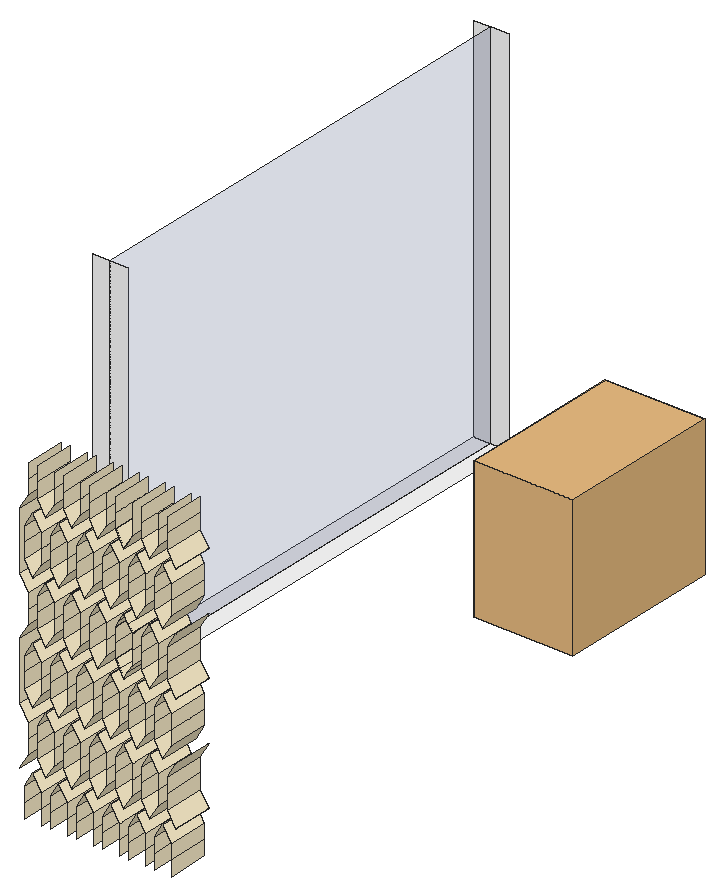
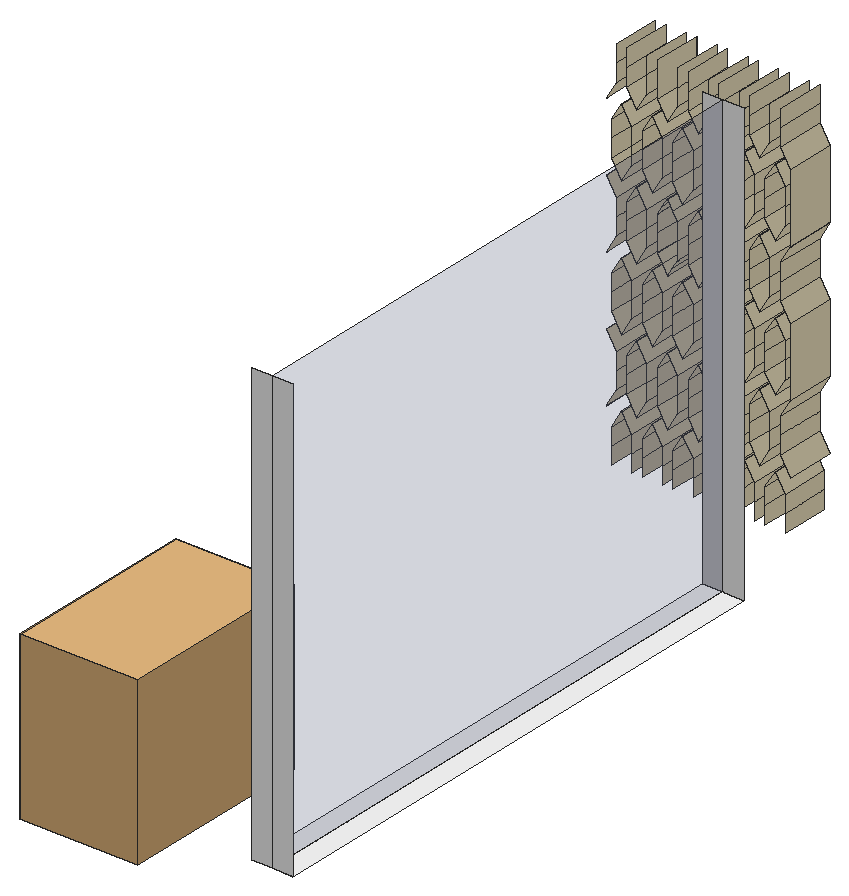
# SketchUp Ruby script. Lengths in inches.
U = 1.inch
M = Sketchup.active_model
def pt(a) = Geom::Point3d.new(a.map { |v| v * U })
def face(e, loops, mat)
  f = e.add_face(loops[0].map { |a| pt(a) })
  loops[1..].each { |l| e.add_face(l.map { |a| pt(a) }).erase! }
  f.material = f.back_material = mat if mat
  f
end
# faces: each face lists its corners as indices into pts; further lists are holes
def faces(e, pts, list, mat = nil) = list.each { |f| face(e, (f[0].is_a?(Array) ? f : [f]).map { |l| l.map { |i| pts[i] } }, mat) }
# xy, xz, yz: faces in a plane at the given z, y or x. An outline is a flat list of corners, or four numbers for a rectangle; further outlines are holes
def ring(l) = l.size == 4 ? [[l[0], l[1]], [l[2], l[1]], [l[2], l[3]], [l[0], l[3]]] : l.each_slice(2).to_a
def flat(e, list, mat, &to3) = list.each { |f| face(e, (f[0].is_a?(Array) ? f : [f]).map { |l| ring(l).map { |u, v| to3.(u, v) } }, mat) }
def xy(e, z, list, mat = nil) = flat(e, list, mat) { |x, y| [x, y, z] }
def xz(e, y, list, mat = nil) = flat(e, list, mat) { |x, z| [x, y, z] }
def yz(e, x, list, mat = nil) = flat(e, list, mat) { |y, z| [x, y, z] }
def lines(e, pts, list) = list.each { |a, b| e.add_line(pt(pts[a]), pt(pts[b])) }
# prism: a flat outline (further loops are holes) pulled along v
def prism(e, loops, v, mat = nil)
  f = face(e, loops, mat); d = Geom::Vector3d.new(v.map { |x| x * U })
  f.pushpull(f.normal.samedirection?(d) ? d.length : -d.length)
end
def box(e, o, s, mat = nil) = prism(e, [[o, [o[0] + s[0], o[1], o[2]], [o[0] + s[0], o[1] + s[1], o[2]], [o[0], o[1] + s[1], o[2]]]], [0, 0, s[2]], mat)
def at(x, y, z, deg = 0) = Geom::Transformation.translation(pt([x, y, z])) * Geom::Transformation.rotation(ORIGIN, Z_AXIS, deg.degrees)
def axes(o, x, y, z) = Geom::Transformation.new([*x, 0, *y, 0, *z, 0, *pt(o).to_a, 1])
def part(name) = M.definitions.add(name)
# library, detail: a bought-in or finely detailed component or shape, given as its bounding box
def library(name, o, s) = part(name).tap { |d| box(d.entities, o, s) }
def detail(e, o, s) = box(e.add_group.entities, o, s)
def put(e, d, t, mat = nil) = e.add_instance(d, t).tap { |i| i.material = mat if mat }
def group(e, t, mat = nil) = e.add_group.tap { |g| g.transformation = t; g.material = mat if mat }.entities
root = M.entities
M.materials.add("D01_Frost_White").color = [255, 242, 206]
M.materials.add("Glass_Sky Reflection_01").color = [126, 138, 183]
M.materials["Glass_Sky Reflection_01"].alpha = 0.25
M.materials.add("M00_Soft_Cloud").color = [255, 255, 255]
c1 = library("FF_Model_ID8636_1_ruthrocker1",[-22.29,-12.06,-2.32],[42.44,25.59,36.01])
xy(root,149.0192,[[126,153.6841,130.5,276.2837],[130.5,153.6841,135,276.2837]],"M00_Soft_Cloud")
xy(root,197.0101,[[183.1657,109.0676,183.1728,119.6039]],"D01_Frost_White")
xy(root,197.0223,[[163.0893,109.0676,163.0964,119.6039],[169.7802,109.0676,169.7874,119.6039]],"D01_Frost_White")
xz(root,109.0676,[[169.7874,182.0245,169.7909,182.0306,168.6907,183.8901],[169.7945,182.0245,170.8947,183.9084,169.7909,182.0306],[168.6907,183.8901,167.5869,185.7679,167.5869,185.7557],[170.8947,183.9084,171.9914,185.774,171.9914,185.7861],[167.5869,185.7679,167.5833,189.5052,167.5833,185.774],
  [171.9914,185.7861,171.995,185.7922,171.9914,189.5416],[167.5833,189.5052,167.5833,193.2607,167.5797,193.2546],[171.9914,189.5416,171.9914,193.2728,171.9879,193.2789],[167.5833,193.2607,168.68,195.1384,167.5833,193.2728],[171.9879,193.2789,171.9878,193.2911,170.884,195.1567],
  [168.68,195.1384,169.7838,197.0162,169.7802,197.0223],[170.884,195.1567,169.7909,197.0162,169.7909,197.0163,169.7874,197.0223,169.7838,197.0162],[183.1639,197.0101,183.1657,197.0101,183.1656,197.0102,183.1639,197.0132],[169.7838,197.0162,169.7874,197.0223,169.7802,197.0223],[143.0236,197.0223,143.0271,197.0224,143.0236,197.0283],
  [143.0236,197.0223,143.0272,197.0223,143.0271,197.0224],[149.711,197.0223,149.7181,197.0223,149.7162,197.0256,149.7129,197.0256],[156.4019,197.0223,156.4055,197.0223,156.4054,197.0224,156.4037,197.0253],[156.4055,197.0223,156.4055,197.0283,156.4037,197.0253,156.4054,197.0224],[149.7129,197.0256,149.7162,197.0256,149.7146,197.0283],
  [183.1639,212.0169,183.1675,212.023,183.1639,212.0291],[169.7802,212.0321,167.5797,215.7876,167.5797,215.7755],[167.5797,215.7876,167.5833,223.2804,167.5797,223.2743]],"D01_Frost_White")
xz(root,153.6841,[[126,149.0192,130.5,245.0192],[130.5,149.0192,135,245.0192]],"M00_Soft_Cloud")
xz(root,276.2837,[[126,149.0192,130.5,245.0192],[130.5,149.0192,135,245.0192]],"M00_Soft_Cloud")
yz(root,130.5,[[153.6841,149.0192,276.2837,245.0192]],"Glass_Sky Reflection_01")
yz(root,143.0236,[[109.0676,167.0329,119.6039,182.0306],[109.0676,197.0283,119.6039,212.0261]],"D01_Frost_White")
yz(root,144.165,[[109.0676,140.7869,119.6039,144.5363],[109.0676,144.5363,119.6039,148.2857],[109.0676,170.7823,119.6039,174.5318],[109.0676,174.5318,119.6039,178.2812],[109.0676,200.7778,119.6039,204.5272],
  [109.0676,204.5272,119.6039,208.2766]],"D01_Frost_White")
yz(root,145.2277,[[109.0676,155.7846,119.6039,159.534],[109.0676,159.534,119.6039,163.2835],[109.0676,185.78,119.6039,189.5295],[109.0676,189.5295,119.6039,193.2789],[109.0676,215.7755,119.6039,219.5249],
  [109.0676,219.5249,119.6039,223.2743]],"D01_Frost_White")
yz(root,147.5105,[[109.0676,155.7846,119.6039,159.534],[109.0676,159.534,119.6039,163.2835],[109.0676,185.78,119.6039,189.5295],[109.0676,189.5295,119.6039,193.2789],[109.0676,215.7755,119.6039,219.5249],
  [109.0676,219.5249,119.6039,223.2743]],"D01_Frost_White")
yz(root,148.5731,[[109.0676,140.7869,119.6039,144.5363],[109.0676,144.5363,119.6039,148.2857],[109.0676,170.7823,119.6039,174.5318],[109.0676,174.5318,119.6039,178.2812],[109.0676,200.7778,119.6039,204.5272],
  [109.0676,204.5272,119.6039,208.2766]],"D01_Frost_White")
yz(root,150.856,[[109.0676,140.7869,119.6039,144.5363],[109.0676,144.5363,119.6039,148.2857],[109.0676,170.7823,119.6039,174.5318],[109.0676,174.5318,119.6039,178.2812],[109.0676,200.7778,119.6039,204.5272],
  [109.0676,204.5272,119.6039,208.2766]],"D01_Frost_White")
yz(root,151.9186,[[109.0676,155.7846,119.6039,159.534],[109.0676,159.534,119.6039,163.2835],[109.0676,185.78,119.6039,189.5295],[109.0676,189.5295,119.6039,193.2789],[109.0676,215.7755,119.6039,219.5249],
  [109.0676,219.5249,119.6039,223.2743]],"D01_Frost_White")
yz(root,154.2015,[[109.0676,155.7846,119.6039,159.534],[109.0676,159.534,119.6039,163.2835],[109.0676,185.78,119.6039,189.5295],[109.0676,189.5295,119.6039,193.2789],[109.0676,215.7755,119.6039,219.5249],
  [109.0676,219.5249,119.6039,223.2743]],"D01_Frost_White")
yz(root,155.2641,[[109.0676,140.7869,119.6039,144.5363],[109.0676,144.5363,119.6039,148.2857],[109.0676,170.7823,119.6039,174.5318],[109.0676,174.5318,119.6039,178.2812],[109.0676,200.7778,119.6039,204.5272],
  [109.0676,204.5272,119.6039,208.2766]],"D01_Frost_White")
yz(root,156.4055,[[109.0676,152.0291,119.6039,152.0352],[109.0676,167.0268,119.6039,167.0329],[109.0676,182.0245,119.6039,182.0306],[109.0676,197.0223,119.6039,197.0283]],"D01_Frost_White")
yz(root,157.5433,[[109.0676,200.7778,119.6039,204.5272],[109.0676,204.5272,119.6039,208.2766]],"D01_Frost_White")
yz(root,157.5469,[[109.0676,140.7808,119.6039,144.5302],[109.0676,144.5302,119.6039,148.2797],[109.0676,170.7762,119.6039,174.5257],[109.0676,174.5257,119.6039,178.2751]],"D01_Frost_White")
yz(root,158.606,[[109.0676,215.7755,119.6039,219.5249],[109.0676,219.5249,119.6039,223.2743]],"D01_Frost_White")
yz(root,158.6095,[[109.0676,155.7785,119.6039,159.528],[109.0676,159.528,119.6039,163.2774],[109.0676,185.774,119.6039,189.5234],[109.0676,189.5234,119.6039,193.2728]],"D01_Frost_White")
yz(root,160.8888,[[109.0676,215.7755,119.6039,219.5249],[109.0676,219.5249,119.6039,223.2743]],"D01_Frost_White")
yz(root,160.8924,[[109.0676,155.7785,119.6039,159.528],[109.0676,159.528,119.6039,163.2774],[109.0676,185.774,119.6039,189.5234],[109.0676,189.5234,119.6039,193.2728]],"D01_Frost_White")
yz(root,161.9514,[[109.0676,200.7778,119.6039,204.5272],[109.0676,204.5272,119.6039,208.2766]],"D01_Frost_White")
yz(root,161.955,[[109.0676,140.7808,119.6039,144.5302],[109.0676,144.5302,119.6039,148.2797],[109.0676,170.7762,119.6039,174.5257],[109.0676,174.5257,119.6039,178.2751]],"D01_Frost_White")
yz(root,164.2343,[[109.0676,200.7778,119.6039,204.5272],[109.0676,204.5272,119.6039,208.2766]],"D01_Frost_White")
yz(root,164.2379,[[109.0676,140.7808,119.6039,144.5302],[109.0676,144.5302,119.6039,148.2797],[109.0676,170.7762,119.6039,174.5257],[109.0676,174.5257,119.6039,178.2751]],"D01_Frost_White")
yz(root,165.2969,[[109.0676,215.7755,119.6039,219.5249],[109.0676,219.5249,119.6039,223.2743]],"D01_Frost_White")
yz(root,165.3005,[[109.0676,155.7785,119.6039,159.528],[109.0676,159.528,119.6039,163.2774],[109.0676,185.774,119.6039,189.5234],[109.0676,189.5234,119.6039,193.2728]],"D01_Frost_White")
yz(root,167.5797,[[109.0676,215.7755,119.6039,215.7876],[109.0676,215.7876,119.6039,219.5249],[109.0676,219.5249,119.6039,223.2743]],"D01_Frost_White")
yz(root,167.5833,[[109.0676,155.7785,119.6039,159.528],[109.0676,159.528,119.6039,163.2774],[109.0676,185.774,119.6039,189.5052],[109.0676,193.2607,119.6039,193.2728]],"D01_Frost_White")
yz(root,167.5869,[[109.0676,185.7557,119.6039,185.7679]],"D01_Frost_White")
yz(root,168.6424,[[109.0676,200.7778,119.6039,204.5272],[109.0676,204.5272,119.6039,208.2766]],"D01_Frost_White")
yz(root,168.6459,[[109.0676,140.7808,119.6039,144.5302],[109.0676,144.5302,119.6039,148.2797],[109.0676,170.7762,119.6039,174.5257],[109.0676,174.5257,119.6039,178.2751]],"D01_Frost_White")
yz(root,169.7909,[[109.0676,197.0162,119.6039,197.0163]],"D01_Frost_White")
yz(root,170.9288,[[109.0676,140.7808,119.6039,144.5302],[109.0676,144.5302,119.6039,148.2797],[109.0676,170.7762,119.6039,174.5257],[109.0676,174.5257,119.6039,178.2751],[109.0676,200.7717,119.6039,204.5211],
  [109.0676,204.5211,119.6039,208.2706]],"D01_Frost_White")
yz(root,171.9914,[[109.0676,155.7785,119.6039,159.528],[109.0676,159.528,119.6039,163.2774],[109.0676,185.774,119.6039,185.7861],[109.0676,189.5416,119.6039,193.2728]],"D01_Frost_White")
yz(root,174.2743,[[109.0676,155.7785,119.6039,159.528],[109.0676,159.528,119.6039,163.2774],[109.0676,185.774,119.6039,189.5234],[109.0676,189.5234,119.6039,193.2728],[109.0676,215.7694,119.6039,219.5188],
  [109.0676,219.5188,119.6039,223.2683]],"D01_Frost_White")
yz(root,175.3369,[[109.0676,140.7808,119.6039,144.5302],[109.0676,144.5302,119.6039,148.2797],[109.0676,170.7762,119.6039,174.5257],[109.0676,174.5257,119.6039,178.2751],[109.0676,200.7717,119.6039,204.5211],
  [109.0676,204.5211,119.6039,208.2706]],"D01_Frost_White")
yz(root,177.6197,[[109.0676,140.7808,119.6039,144.5302],[109.0676,144.5302,119.6039,148.2797],[109.0676,170.7762,119.6039,174.5257],[109.0676,174.5257,119.6039,178.2751],[109.0676,200.7717,119.6039,204.5211],
  [109.0676,204.5211,119.6039,208.2706]],"D01_Frost_White")
yz(root,178.6824,[[109.0676,155.7785,119.6039,159.528],[109.0676,159.528,119.6039,163.2774],[109.0676,185.774,119.6039,189.5234],[109.0676,189.5234,119.6039,193.2728],[109.0676,215.7694,119.6039,219.5188],
  [109.0676,219.5188,119.6039,223.2683]],"D01_Frost_White")
yz(root,180.9652,[[109.0676,155.7785,119.6039,159.528],[109.0676,159.528,119.6039,163.2774],[109.0676,185.774,119.6039,189.5234],[109.0676,189.5234,119.6039,193.2728],[109.0676,215.7694,119.6039,219.5188],
  [109.0676,219.5188,119.6039,223.2683]],"D01_Frost_White")
yz(root,182.0278,[[109.0676,140.7808,119.6039,144.5302],[109.0676,144.5302,119.6039,148.2797],[109.0676,170.7762,119.6039,174.5257],[109.0676,174.5257,119.6039,178.2751],[109.0676,200.7717,119.6039,204.5211],
  [109.0676,204.5211,119.6039,208.2706]],"D01_Frost_White")
yz(root,183.1639,[[109.0676,212.0169,119.6039,212.0291]],"D01_Frost_White")
yz(root,183.1692,[[109.0676,152.023,119.6039,152.0291],[109.0676,167.0207,119.6039,167.0268],[109.0676,182.0185,119.6039,182.0245]],"D01_Frost_White")
p = [[144.165,109.0676,148.2857],[146.3691,109.0676,152.0352],[146.3691,119.6039,152.0352],[144.165,119.6039,148.2857],[148.5731,109.0676,148.2857],[148.5731,119.6039,148.2857],
  [150.856,109.0676,148.2857],[153.06,109.0676,152.0352],[153.06,119.6039,152.0352],[150.856,119.6039,148.2857],[155.2641,109.0676,148.2857],[155.2641,119.6039,148.2857],
  [157.5469,109.0676,148.2797],[159.751,109.0676,152.0291],[159.751,119.6039,152.0291],[157.5469,119.6039,148.2797],[161.955,109.0676,148.2797],[161.955,119.6039,148.2797],
  [164.2379,109.0676,148.2797],[166.4419,109.0676,152.0291],[166.4419,119.6039,152.0291],[164.2379,119.6039,148.2797],[168.6459,109.0676,148.2797],[168.6459,119.6039,148.2797],
  [170.9288,109.0676,148.2797],[173.1328,109.0676,152.0291],[173.1328,119.6039,152.0291],[170.9288,119.6039,148.2797],[175.3369,109.0676,148.2797],[175.3369,119.6039,148.2797],
  [177.6197,109.0676,148.2797],[179.8238,109.0676,152.0291],[179.8238,119.6039,152.0291],[177.6197,119.6039,148.2797],[182.0278,109.0676,148.2797],[182.0278,119.6039,148.2797],
  [145.2277,109.0676,155.7846],[143.0236,109.0676,152.0352],[143.0236,119.6039,152.0352],[145.2277,119.6039,155.7846],[149.7146,109.0676,152.0352],[147.5105,109.0676,155.7846],
  [147.5105,119.6039,155.7846],[149.7146,119.6039,152.0352],[151.9186,109.0676,155.7846],[151.9186,119.6039,155.7846],[156.4055,109.0676,152.0352],[154.2015,109.0676,155.7846],
  [154.2015,119.6039,155.7846],[156.4055,119.6039,152.0352],[158.6095,109.0676,155.7785],[156.4055,109.0676,152.0291],[156.4055,119.6039,152.0291],[158.6095,119.6039,155.7785],
  [163.0964,109.0676,152.0291],[160.8924,109.0676,155.7785],[160.8924,119.6039,155.7785],[163.0964,119.6039,152.0291],[165.3005,109.0676,155.7785],[165.3005,119.6039,155.7785],
  [169.7874,109.0676,152.0291],[167.5833,109.0676,155.7785],[167.5833,119.6039,155.7785],[169.7874,119.6039,152.0291],[171.9914,109.0676,155.7785],[171.9914,119.6039,155.7785],
  [176.4783,109.0676,152.0291],[174.2743,109.0676,155.7785],[174.2743,119.6039,155.7785],[176.4783,119.6039,152.0291],[178.6824,109.0676,155.7785],[178.6824,119.6039,155.7785],
  [183.1692,109.0676,152.0291],[180.9652,109.0676,155.7785],[180.9652,119.6039,155.7785],[183.1692,119.6039,152.0291],[143.0236,109.0676,167.0329],[145.2277,109.0676,163.2835],
  [145.2277,119.6039,163.2835],[143.0236,119.6039,167.0329],[147.5105,109.0676,163.2835],[149.7146,109.0676,167.0329],[149.7146,119.6039,167.0329],[147.5105,119.6039,163.2835],
  [151.9186,109.0676,163.2835],[151.9186,119.6039,163.2835],[154.2015,109.0676,163.2835],[156.4055,109.0676,167.0329],[156.4055,119.6039,167.0329],[154.2015,119.6039,163.2835],
  [156.4055,109.0676,167.0268],[158.6095,109.0676,163.2774],[158.6095,119.6039,163.2774],[156.4055,119.6039,167.0268],[160.8924,109.0676,163.2774],[163.0964,109.0676,167.0268],
  [163.0964,119.6039,167.0268],[160.8924,119.6039,163.2774],[165.3005,109.0676,163.2774],[165.3005,119.6039,163.2774],[167.5833,109.0676,163.2774],[169.7874,109.0676,167.0268],
  [169.7874,119.6039,167.0268],[167.5833,119.6039,163.2774],[171.9914,109.0676,163.2774],[171.9914,119.6039,163.2774],[174.2743,109.0676,163.2774],[176.4783,109.0676,167.0268],
  [176.4783,119.6039,167.0268],[174.2743,119.6039,163.2774],[178.6824,109.0676,163.2774],[178.6824,119.6039,163.2774],[180.9652,109.0676,163.2774],[183.1692,109.0676,167.0268],
  [183.1692,119.6039,167.0268],[180.9652,119.6039,163.2774],[146.3691,109.0676,167.0329],[144.165,109.0676,170.7823],[144.165,119.6039,170.7823],[146.3691,119.6039,167.0329],
  [148.5731,109.0676,170.7823],[148.5731,119.6039,170.7823],[153.06,109.0676,167.0329],[150.856,109.0676,170.7823],[150.856,119.6039,170.7823],[153.06,119.6039,167.0329],
  [155.2641,109.0676,170.7823],[155.2641,119.6039,170.7823],[159.751,109.0676,167.0268],[157.5469,109.0676,170.7762],[157.5469,119.6039,170.7762],[159.751,119.6039,167.0268],
  [161.955,109.0676,170.7762],[161.955,119.6039,170.7762],[166.4419,109.0676,167.0268],[164.2379,109.0676,170.7762],[164.2379,119.6039,170.7762],[166.4419,119.6039,167.0268],
  [168.6459,109.0676,170.7762],[168.6459,119.6039,170.7762],[173.1328,109.0676,167.0268],[170.9288,109.0676,170.7762],[170.9288,119.6039,170.7762],[173.1328,119.6039,167.0268],
  [175.3369,109.0676,170.7762],[175.3369,119.6039,170.7762],[179.8238,109.0676,167.0268],[177.6197,109.0676,170.7762],[177.6197,119.6039,170.7762],[179.8238,119.6039,167.0268],
  [182.0278,109.0676,170.7762],[182.0278,119.6039,170.7762],[144.165,109.0676,178.2812],[146.3691,109.0676,182.0306],[146.3691,119.6039,182.0306],[144.165,119.6039,178.2812],
  [148.5731,109.0676,178.2812],[148.5731,119.6039,178.2812],[150.856,109.0676,178.2812],[153.06,109.0676,182.0306],[153.06,119.6039,182.0306],[150.856,119.6039,178.2812],
  [155.2641,109.0676,178.2812],[155.2641,119.6039,178.2812],[157.5469,109.0676,178.2751],[159.751,109.0676,182.0245],[159.751,119.6039,182.0245],[157.5469,119.6039,178.2751],
  [161.955,109.0676,178.2751],[161.955,119.6039,178.2751],[164.2379,109.0676,178.2751],[166.4419,109.0676,182.0245],[166.4419,119.6039,182.0245],[164.2379,119.6039,178.2751],
  [168.6459,109.0676,178.2751],[168.6459,119.6039,178.2751],[170.9288,109.0676,178.2751],[173.1328,109.0676,182.0245],[173.1328,119.6039,182.0245],[170.9288,119.6039,178.2751],
  [175.3369,109.0676,178.2751],[175.3369,119.6039,178.2751],[177.6197,109.0676,178.2751],[179.8238,109.0676,182.0245],[179.8238,119.6039,182.0245],[177.6197,119.6039,178.2751],
  [182.0278,109.0676,178.2751],[182.0278,119.6039,178.2751],[145.2277,109.0676,185.78],[143.0236,109.0676,182.0306],[143.0236,119.6039,182.0306],[145.2277,119.6039,185.78],
  [149.7146,109.0676,182.0306],[147.5105,109.0676,185.78],[147.5105,119.6039,185.78],[149.7146,119.6039,182.0306],[151.9186,109.0676,185.78],[151.9186,119.6039,185.78],
  [156.4055,109.0676,182.0306],[154.2015,109.0676,185.78],[154.2015,119.6039,185.78],[156.4055,119.6039,182.0306],[158.6095,109.0676,185.774],[156.4055,109.0676,182.0245],
  [156.4055,119.6039,182.0245],[158.6095,119.6039,185.774],[163.0964,109.0676,182.0245],[160.8924,109.0676,185.774],[160.8924,119.6039,185.774],[163.0964,119.6039,182.0245],
  [165.3005,109.0676,185.774],[165.3005,119.6039,185.774],[169.7874,109.0676,182.0245],[168.6907,109.0676,183.8901],[168.6907,119.6039,183.8901],[169.7874,119.6039,182.0245],
  [169.7909,109.0676,182.0306],[169.7909,119.6039,182.0306],[169.7945,109.0676,182.0245],[169.7945,119.6039,182.0245],[170.8947,109.0676,183.9084],[170.8947,119.6039,183.9084],
  [176.4783,109.0676,182.0245],[174.2743,109.0676,185.774],[174.2743,119.6039,185.774],[176.4783,119.6039,182.0245],[178.6824,109.0676,185.774],[178.6824,119.6039,185.774],
  [183.1692,109.0676,182.0245],[180.9652,109.0676,185.774],[180.9652,119.6039,185.774],[183.1692,119.6039,182.0245],[167.5869,109.0676,185.7557],[167.5869,119.6039,185.7557],
  [171.9914,109.0676,185.774],[171.9914,119.6039,185.774],[167.5869,109.0676,185.7679],[167.5833,109.0676,185.774],[167.5833,119.6039,185.774],[167.5869,119.6039,185.7679],
  [171.9914,109.0676,189.5416],[171.995,109.0676,185.7922],[171.995,119.6039,185.7922],[171.9914,119.6039,189.5416],[171.9914,109.0676,185.7861],[171.9914,119.6039,185.7861],
  [167.5833,109.0676,189.5052],[167.5797,109.0676,193.2546],[167.5797,119.6039,193.2546],[167.5833,119.6039,189.5052],[143.0272,109.0676,197.0223],[145.2277,109.0676,193.2789],
  [145.2277,119.6039,193.2789],[143.0272,119.6039,197.0223],[147.5105,109.0676,193.2789],[149.711,109.0676,197.0223],[149.711,119.6039,197.0223],[147.5105,119.6039,193.2789],
  [149.7181,109.0676,197.0223],[151.9186,109.0676,193.2789],[151.9186,119.6039,193.2789],[149.7181,119.6039,197.0223],[154.2015,109.0676,193.2789],[156.4019,109.0676,197.0223],
  [156.4019,119.6039,197.0223],[154.2015,119.6039,193.2789],[156.4055,109.0676,197.0223],[158.6095,109.0676,193.2728],[158.6095,119.6039,193.2728],[156.4055,119.6039,197.0223],
  [160.8924,109.0676,193.2728],[163.0964,109.0676,197.0223],[163.0964,119.6039,197.0223],[160.8924,119.6039,193.2728],[165.3005,109.0676,193.2728],[165.3005,119.6039,193.2728],
  [167.5833,109.0676,193.2607],[167.5833,119.6039,193.2607],[167.5833,109.0676,193.2728],[168.68,109.0676,195.1384],[168.68,119.6039,195.1384],[167.5833,119.6039,193.2728],
  [170.884,109.0676,195.1567],[171.9878,109.0676,193.2911],[171.9878,119.6039,193.2911],[170.884,119.6039,195.1567],[171.9879,109.0676,193.2789],[171.9879,119.6039,193.2789],
  [171.9914,109.0676,193.2728],[171.9914,119.6039,193.2728],[174.2743,109.0676,193.2728],[176.4747,109.0676,197.0162],[176.4747,119.6039,197.0162],[174.2743,119.6039,193.2728],
  [176.4819,109.0676,197.0162],[178.6824,109.0676,193.2728],[178.6824,119.6039,193.2728],[176.4819,119.6039,197.0162],[180.9652,109.0676,193.2728],[183.1639,109.0676,197.0132],
  [183.1639,119.6039,197.0132],[180.9652,119.6039,193.2728],[169.7802,109.0676,197.0223],[169.7802,119.6039,197.0223],[169.7909,109.0676,197.0162],[169.7909,119.6039,197.0162],
  [143.0236,109.0676,197.0283],[143.0271,109.0676,197.0224],[143.0271,119.6039,197.0224],[143.0236,119.6039,197.0283],[146.3691,109.0676,197.0283],[144.165,109.0676,200.7778],
  [144.165,119.6039,200.7778],[146.3691,119.6039,197.0283],[148.5731,109.0676,200.7778],[148.5731,119.6039,200.7778],[149.7129,109.0676,197.0256],[149.7129,119.6039,197.0256],
  [149.7146,109.0676,197.0283],[149.7146,119.6039,197.0283],[149.7162,109.0676,197.0256],[149.7162,119.6039,197.0256],[153.06,109.0676,197.0283],[150.856,109.0676,200.7778],
  [150.856,119.6039,200.7778],[153.06,119.6039,197.0283],[155.2641,109.0676,200.7778],[155.2641,119.6039,200.7778],[156.4037,109.0676,197.0253],[156.4037,119.6039,197.0253],
  [156.4055,109.0676,197.0283],[156.4055,119.6039,197.0283],[159.7474,109.0676,197.0283],[157.5433,109.0676,200.7778],[157.5433,119.6039,200.7778],[159.7474,119.6039,197.0283],
  [161.9514,109.0676,200.7778],[161.9514,119.6039,200.7778],[163.0893,109.0676,197.0223],[163.0912,109.0676,197.0256],[163.0912,119.6039,197.0256],[163.0893,119.6039,197.0223],
  [163.0929,109.0676,197.0283],[163.0929,119.6039,197.0283],[163.0945,109.0676,197.0256],[163.0945,119.6039,197.0256],[166.4383,109.0676,197.0283],[164.2343,109.0676,200.7778],
  [164.2343,119.6039,200.7778],[166.4383,119.6039,197.0283],[168.6424,109.0676,200.7778],[168.6424,119.6039,200.7778],[169.7874,109.0676,197.0223],[169.7909,109.0676,197.0163],
  [169.7909,119.6039,197.0163],[169.7874,119.6039,197.0223],[173.1328,109.0676,197.0223],[170.9288,109.0676,200.7717],[170.9288,119.6039,200.7717],[173.1328,119.6039,197.0223],
  [175.3369,109.0676,200.7717],[175.3369,119.6039,200.7717],[176.4767,109.0676,197.0195],[176.4767,119.6039,197.0195],[176.4783,109.0676,197.0223],[176.4783,119.6039,197.0223],
  [176.4799,109.0676,197.0195],[176.4799,119.6039,197.0195],[179.8238,109.0676,197.0223],[177.6197,109.0676,200.7717],[177.6197,119.6039,200.7717],[179.8238,119.6039,197.0223],
  [182.0278,109.0676,200.7717],[182.0278,119.6039,200.7717],[183.1656,109.0676,197.0102],[183.1656,119.6039,197.0102],[183.1657,109.0676,197.0101],[183.1657,119.6039,197.0101],
  [144.165,109.0676,208.2766],[146.3691,109.0676,212.0261],[146.3691,119.6039,212.0261],[144.165,119.6039,208.2766],[148.5731,109.0676,208.2766],[148.5731,119.6039,208.2766],
  [150.856,109.0676,208.2766],[153.06,109.0676,212.0261],[153.06,119.6039,212.0261],[150.856,119.6039,208.2766],[155.2641,109.0676,208.2766],[155.2641,119.6039,208.2766],
  [157.5433,109.0676,208.2766],[159.7474,109.0676,212.0261],[159.7474,119.6039,212.0261],[157.5433,119.6039,208.2766],[161.9514,109.0676,208.2766],[161.9514,119.6039,208.2766],
  [164.2343,109.0676,208.2766],[166.4383,109.0676,212.0261],[166.4383,119.6039,212.0261],[164.2343,119.6039,208.2766],[168.6424,109.0676,208.2766],[168.6424,119.6039,208.2766],
  [170.9288,109.0676,208.2706],[173.1328,109.0676,212.02],[173.1328,119.6039,212.02],[170.9288,119.6039,208.2706],[175.3369,109.0676,208.2706],[175.3369,119.6039,208.2706],
  [177.6197,109.0676,208.2706],[179.8238,109.0676,212.02],[179.8238,119.6039,212.02],[177.6197,119.6039,208.2706],[182.0278,109.0676,208.2706],[182.0278,119.6039,208.2706],
  [145.2277,109.0676,215.7755],[143.0236,109.0676,212.0261],[143.0236,119.6039,212.0261],[145.2277,119.6039,215.7755],[149.7146,109.0676,212.0261],[147.5105,109.0676,215.7755],
  [147.5105,119.6039,215.7755],[149.7146,119.6039,212.0261],[151.9186,109.0676,215.7755],[151.9186,119.6039,215.7755],[156.4037,109.0676,212.0291],[154.2015,109.0676,215.7755],
  [154.2015,119.6039,215.7755],[156.4037,119.6039,212.0291],[158.606,109.0676,215.7755],[158.606,119.6039,215.7755],[163.0929,109.0676,212.0261],[160.8888,109.0676,215.7755],
  [160.8888,119.6039,215.7755],[163.0929,119.6039,212.0261],[165.2969,109.0676,215.7755],[165.2969,119.6039,215.7755],[169.7802,109.0676,212.0321],[167.5797,109.0676,215.7755],
  [167.5797,119.6039,215.7755],[169.7802,119.6039,212.0321],[171.9843,109.0676,215.7694],[171.9843,119.6039,215.7694],[176.4783,109.0676,212.02],[174.2743,109.0676,215.7694],
  [174.2743,119.6039,215.7694],[176.4783,119.6039,212.02],[178.6824,109.0676,215.7694],[178.6824,119.6039,215.7694],[183.1639,109.0676,212.0291],[180.9652,109.0676,215.7694],
  [180.9652,119.6039,215.7694],[183.1639,119.6039,212.0291],[183.1675,109.0676,212.023],[183.1639,109.0676,212.0169],[183.1639,119.6039,212.0169],[183.1675,119.6039,212.023],
  [171.9878,109.0676,223.2622],[171.9878,119.6039,223.2622],[183.1692,109.0676,197.0162],[183.1728,109.0676,197.0101],[183.1657,109.0676,197.0162],[183.1692,109.0676,197.0223],
  [183.1692,109.0676,212.02],[183.1621,109.0676,212.0139],[169.7838,109.0676,212.0261],[169.7838,109.0676,197.0283],[153.06,109.0676,197.0223],[146.3691,109.0676,197.0223],
  [171.9914,109.0676,223.2683],[171.9914,109.0676,219.5188],[171.9914,109.0676,215.7694],[169.7874,109.0676,212.02],[156.4055,109.0676,212.0261],[183.1621,109.0676,197.0162],
  [156.4019,109.0676,212.0261],[156.4019,109.0676,197.0283]]
faces(root,p,[[0,1,2,3],[1,4,5,2],[6,7,8,9],[7,10,11,8],[12,13,14,15],[13,16,17,14],[18,19,20,21],[19,22,23,20],
  [24,25,26,27],[25,28,29,26],[30,31,32,33],[31,34,35,32],[36,37,38,39],[40,41,42,43],[44,40,43,45],[46,47,48,49],
  [50,51,52,53],[54,55,56,57],[58,54,57,59],[60,61,62,63],[64,60,63,65],[66,67,68,69],[70,66,69,71],[72,73,74,75],
  [76,77,78,79],[80,81,82,83],[81,84,85,82],[86,87,88,89],[90,91,92,93],[94,95,96,97],[95,98,99,96],[100,101,102,103],
  [101,104,105,102],[106,107,108,109],[107,110,111,108],[112,113,114,115],[116,117,118,119],[120,116,119,121],[122,123,124,125],[126,122,125,127],
  [128,129,130,131],[132,128,131,133],[134,135,136,137],[138,134,137,139],[140,141,142,143],[144,140,143,145],[146,147,148,149],[150,146,149,151],
  [152,153,154,155],[153,156,157,154],[158,159,160,161],[159,162,163,160],[164,165,166,167],[165,168,169,166],[170,171,172,173],[171,174,175,172],
  [176,177,178,179],[177,180,181,178],[182,183,184,185],[183,186,187,184],[188,189,190,191],[192,193,194,195],[196,192,195,197],[198,199,200,201],
  [202,203,204,205],[206,207,208,209],[210,206,209,211],[212,213,214,215],[216,212,215,217],[218,216,217,219],[220,218,219,221],[222,223,224,225],
  [226,222,225,227],[228,229,230,231],[213,232,233,214],[234,220,221,235],[236,237,238,239],[240,241,242,243],[241,244,245,242],[246,247,248,249],
  [250,251,252,253],[254,255,256,257],[258,259,260,261],[262,263,264,265],[266,267,268,269],[270,271,272,273],[271,274,275,272],[247,276,277,248],
  [278,279,280,281],[282,283,284,285],[283,286,287,284],[286,288,289,287],[290,291,292,293],[294,295,296,297],[298,299,300,301],[279,302,303,280],
  [304,282,285,305],[306,307,308,309],[307,250,253,308],[310,311,312,313],[314,310,313,315],[255,316,317,256],[316,318,319,317],[318,320,321,319],
  [320,258,261,321],[322,323,324,325],[326,322,325,327],[263,328,329,264],[328,330,331,329],[332,333,334,335],[336,332,335,337],[338,339,340,341],
  [339,342,343,340],[342,344,345,343],[344,271,272,345],[346,347,348,349],[350,346,349,351],[352,353,354,355],[356,357,358,359],[360,356,359,361],
  [291,362,363,292],[362,364,365,363],[364,366,367,365],[366,294,297,367],[368,369,370,371],[372,368,371,373],[299,374,375,300],[374,376,377,375],
  [378,379,380,381],[379,382,383,380],[384,385,386,387],[385,388,389,386],[390,391,392,393],[391,394,395,392],[396,397,398,399],[397,400,401,398],
  [402,403,404,405],[403,406,407,404],[408,409,410,411],[409,412,413,410],[414,415,416,417],[418,419,420,421],[422,418,421,423],[424,425,426,427],
  [428,424,427,429],[430,431,432,433],[434,430,433,435],[436,437,438,439],[440,436,439,441],[442,443,444,445],[446,442,445,447],[448,449,450,451],
  [452,453,454,455],[456,440,441,457]],"D01_Frost_White")
lines(root,p,[[458,459],[460,461],[462,452],[453,463],[464,436],[302,465],[299,460],[322,466],[310,467],[468,469],[469,470],[470,471],
  [472,424],[473,299],[424,474],[475,328]])
put(root,c1,at(172.66,253.1,141.02,-90))
